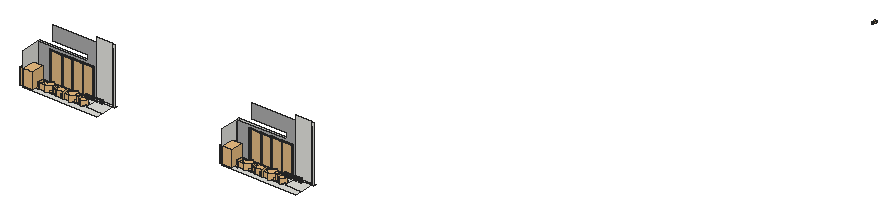
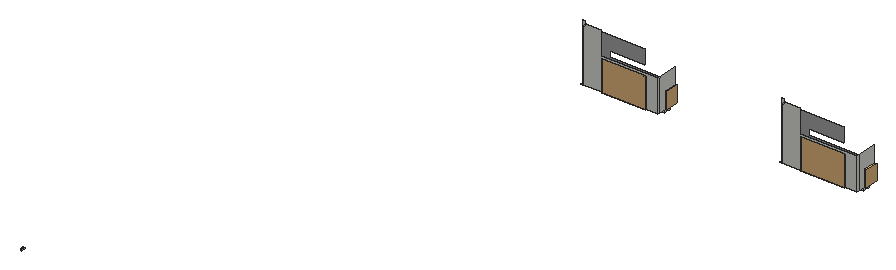
# SketchUp Ruby script. Lengths in inches.
U = 1.inch
M = Sketchup.active_model
def pt(a) = Geom::Point3d.new(a.map { |v| v * U })
def face(e, loops, mat)
  f = e.add_face(loops[0].map { |a| pt(a) })
  loops[1..].each { |l| e.add_face(l.map { |a| pt(a) }).erase! }
  f.material = f.back_material = mat if mat
  f
end
# faces: each face lists its corners as indices into pts; further lists are holes
def faces(e, pts, list, mat = nil) = list.each { |f| face(e, (f[0].is_a?(Array) ? f : [f]).map { |l| l.map { |i| pts[i] } }, mat) }
# xy, xz, yz: faces in a plane at the given z, y or x. An outline is a flat list of corners, or four numbers for a rectangle; further outlines are holes
def ring(l) = l.size == 4 ? [[l[0], l[1]], [l[2], l[1]], [l[2], l[3]], [l[0], l[3]]] : l.each_slice(2).to_a
def flat(e, list, mat, &to3) = list.each { |f| face(e, (f[0].is_a?(Array) ? f : [f]).map { |l| ring(l).map { |u, v| to3.(u, v) } }, mat) }
def xy(e, z, list, mat = nil) = flat(e, list, mat) { |x, y| [x, y, z] }
def xz(e, y, list, mat = nil) = flat(e, list, mat) { |x, z| [x, y, z] }
def yz(e, x, list, mat = nil) = flat(e, list, mat) { |y, z| [x, y, z] }
def lines(e, pts, list) = list.each { |a, b| e.add_line(pt(pts[a]), pt(pts[b])) }
# prism: a flat outline (further loops are holes) pulled along v
def prism(e, loops, v, mat = nil)
  f = face(e, loops, mat); d = Geom::Vector3d.new(v.map { |x| x * U })
  f.pushpull(f.normal.samedirection?(d) ? d.length : -d.length)
end
def box(e, o, s, mat = nil) = prism(e, [[o, [o[0] + s[0], o[1], o[2]], [o[0] + s[0], o[1] + s[1], o[2]], [o[0], o[1] + s[1], o[2]]]], [0, 0, s[2]], mat)
def at(x, y, z, deg = 0) = Geom::Transformation.translation(pt([x, y, z])) * Geom::Transformation.rotation(ORIGIN, Z_AXIS, deg.degrees)
def axes(o, x, y, z) = Geom::Transformation.new([*x, 0, *y, 0, *z, 0, *pt(o).to_a, 1])
def part(name) = M.definitions.add(name)
# library, detail: a bought-in or finely detailed component or shape, given as its bounding box
def library(name, o, s) = part(name).tap { |d| box(d.entities, o, s) }
def detail(e, o, s) = box(e.add_group.entities, o, s)
def put(e, d, t, mat = nil) = e.add_instance(d, t).tap { |i| i.material = mat if mat }
def group(e, t, mat = nil) = e.add_group.tap { |g| g.transformation = t; g.material = mat if mat }.entities
root = M.entities
M.materials.add("Glazing").color = [128, 128, 128]
M.materials["Glazing"].alpha = 0.05
M.materials.add("Material__1").color = [95, 70, 46]
M.materials.add("Powdercoating").color = [41, 44, 40]
M.materials.add("[Color M03]1").color = [170, 170, 170]
c1 = library("plant (1)",[-35.72,-28.42,0],[66.31,67.39,84.38])
c2 = library("Areca palm plant",[0,0,0],[49.1,36.6,54.46])
c3 = library("Group\#589",[-84.69,-90.07,-0.36],[176.51,175.13,171.4])
c4 = library("Group20\#1",[-20.81,-17.08,3.79],[39.86,39.43,37.51])
c5 = library("Group38\#1",[14.01,28.44,-23.43],[18.58,18.32,38.89])
c6 = library("Group\#590",[-7.34,-1.2,0],[38.67,35.81,49.04])
c7 = part("Group\#592")
put(c7.entities,c2,axes([-6.2,56.6,6.08],[0.45017,-0.56191,0],[0.66137,0.52986,0],[0,0,0.72]))
put(c7.entities,c2,axes([-6.2,158.41,6.08],[0.45017,-0.56191,0],[0.66137,0.52986,0],[0,0,0.72]))
put(c7.entities,c3,axes([17.19,15.79,6.07],[-0.08133,-0.14087,0],[0.14087,-0.08133,0],[0,0,0.1725]))
put(c7.entities,c4,axes([18.97,79.98,4.77],[0,0.85,0],[-0.85,0,0],[0,0,0.85]))
put(c7.entities,c5,axes([-4.1,-1.15,28.17],[0.8848,0,0],[0,0.94674,0],[0,0,0.85826]))
put(c7.entities,c3,axes([17.19,121.23,6.07],[-0.08133,-0.14087,0],[0.14087,-0.08133,0],[0,0,0.1725]))
put(c7.entities,c3,axes([14.93,91.37,6.05],[-0.04961,-0.08593,0],[0.08593,-0.04961,0],[0,0,0.10522]))
put(c7.entities,c4,axes([18.97,181.79,4.77],[0,0.85,0],[-0.85,0,0],[0,0,0.85]))
put(c7.entities,c3,axes([14.93,193.18,6.05],[-0.04961,-0.08593,0],[0.08593,-0.04961,0],[0,0,0.10522]))
put(c7.entities,c5,axes([-4.1,100.66,28.17],[0.8848,0,0],[0,0.94674,0],[0,0,0.85826]))
g1 = group(c7.entities,at(0,0,0))
xy(g1,0,[[0,0,6,234.8],[30,0,36,234.8]])
xy(g1,3,[[6,0,30,234.8]])
xy(g1,7,[[6,5,30,229.8]],"Material__1")
xy(g1,15,[[[0,0,36,234.8],[6,5,30,229.8]]])
xz(g1,0,[[0,0,6,0,6,3,30,3,30,0,36,0,36,15,0,15]])
xz(g1,5,[[6,7,30,15]])
xz(g1,229.8,[[6,7,30,15]])
xz(g1,234.8,[[0,0,0,15,36,15,36,0,30,0,30,3,6,3,6,0]])
yz(g1,0,[[0,0,234.8,15]])
yz(g1,6,[[0,0,234.8,3],[5,7,229.8,15]])
yz(g1,30,[[0,0,234.8,3],[5,7,229.8,15]])
yz(g1,36,[[0,0,234.8,15]])
put(c7.entities,c3,axes([17.19,223.04,6.07],[-0.08133,-0.14087,0],[0.14087,-0.08133,0],[0,0,0.1725]))
put(c7.entities,c3,axes([14.93,44.05,6.05],[-0.04961,-0.08593,0],[0.08593,-0.04961,0],[0,0,0.10522]))
put(c7.entities,c3,axes([14.93,173.12,6.05],[-0.04961,-0.08593,0],[0.08593,-0.04961,0],[0,0,0.10522]))
put(c7.entities,c3,axes([14.93,145.87,6.05],[-0.04961,-0.08593,0],[0.08593,-0.04961,0],[0,0,0.10522]))
put(c7.entities,c6,axes([24.9375,89.91,8],[0,0.79,0],[-0.79,0,0],[0,0,0.79]))
put(c7.entities,c3,axes([14.93,71.3,6.05],[-0.04961,-0.08593,0],[0.08593,-0.04961,0],[0,0,0.10522]))
put(c7.entities,c6,axes([24.9375,191.72,8],[0,0.79,0],[-0.79,0,0],[0,0,0.79]))
c8 = part("Group\#15")
xy(c8.entities,0,[[0,-55.94,0.71,45.94]])
xy(c8.entities,0.2,[[0,-55.94,0.47,45.94],[0.47,45.94,0.71,46.42]])
xy(c8.entities,2.36,[[0.47,-55.94,0.71,46.42]])
xz(c8.entities,-55.94,[[0,0,0.71,0,0.71,2.36,0.47,2.36,0.47,0.2,0,0.2]])
xz(c8.entities,45.94,[[0,0,0.71,0.2]])
xz(c8.entities,46.42,[[0.47,0.2,0.71,2.36]])
yz(c8.entities,0,[[-55.94,0,45.94,0.2]])
yz(c8.entities,0.47,[[-55.94,0.2,46.42,2.36]])
yz(c8.entities,0.71,[[-55.94,0,45.94,0,45.94,0.2,46.42,0.2,46.42,2.36,-55.94,2.36]])
c9 = part("Group\#7")
xy(c9.entities,0,[[0,-59.09,0.71,45.94]])
xy(c9.entities,0.2,[[0,-59.09,0.47,45.94],[0.47,45.94,0.71,46.42]])
xy(c9.entities,2.36,[[0.47,-59.09,0.71,46.42]])
xz(c9.entities,-59.09,[[0,0,0.71,0,0.71,2.36,0.47,2.36,0.47,0.2,0,0.2]])
xz(c9.entities,45.94,[[0,0,0.71,0.2]])
xz(c9.entities,46.42,[[0.47,0.2,0.71,2.36]])
yz(c9.entities,0,[[-59.09,0,45.94,0.2]])
yz(c9.entities,0.47,[[-59.09,0.2,46.42,2.36]])
yz(c9.entities,0.71,[[-59.09,0,45.94,0,45.94,0.2,46.42,0.2,46.42,2.36,-59.09,2.36]])
c10 = part("Group\#16")
prism(c10.entities,[[[0.47,-56.18,0.2],[0,-56.18,0.2],[0,-56.18,0],[0.71,-56.18,0],[0.71,-56.18,2.36],[0.47,-56.18,2.36]]],[0,28.68,0])
c11 = part("Group\#10")
box(c11.entities,[-0.73,0,0],[27.99,0.55,102.05])
c12 = part("Group\#18")
xy(c12.entities,0,[[0.47,-56.18,0.47,-55.47,0,-55.47,0,-28.21,1.18,-28.21,1.18,-56.18]])
xy(c12.entities,0.2,[[0.71,-56.18,1.18,-28.21],[0,-55.47,0.47,-28.21],[0.47,-28.21,0.71,-27.74]])
xy(c12.entities,2.36,[[0.47,-56.18,0.71,-27.74]])
xz(c12.entities,-56.18,[[0.47,0,1.18,0,1.18,0.2,0.71,0.2,0.71,2.36,0.47,2.36]])
xz(c12.entities,-55.47,[[0,0,0.47,0.2]])
xz(c12.entities,-28.21,[[0,0,1.18,0.2]])
xz(c12.entities,-27.74,[[0.47,0.2,0.71,2.36]])
yz(c12.entities,0,[[-55.47,0,-28.21,0.2]])
yz(c12.entities,0.47,[[-56.18,0,-55.47,0.2],[-56.18,0.2,-27.74,2.36]])
yz(c12.entities,0.71,[[-56.18,0.2,-27.74,2.36]])
yz(c12.entities,1.18,[[-56.18,0,-28.21,0.2]])
c13 = part("Group\#34")
xy(c13.entities,0,[[-20.45,0,7.76,1.22]])
xy(c13.entities,0.06,[[-20.39,0.06,7.7,1.22]])
xy(c13.entities,0.47,[[-19.98,0,7.28,0.06]])
xy(c13.entities,101.89,[[-19.98,0,7.28,0.06]])
xy(c13.entities,102.3,[[-20.39,0.06,7.7,1.22]])
xy(c13.entities,102.36,[[-20.45,0,7.76,1.22]])
xz(c13.entities,0,[[[-20.45,0,7.76,102.36],[-19.98,0.47,7.28,101.89]]])
xz(c13.entities,0.06,[[[-20.39,0.06,7.7,102.3],[-19.98,0.47,7.28,101.89]]])
xz(c13.entities,1.22,[[[-20.45,0,7.76,102.36],[-20.39,0.06,7.7,102.3]]])
yz(c13.entities,-20.45,[[0,0,1.22,102.36]])
yz(c13.entities,-20.39,[[0.06,0.06,1.22,102.3]])
yz(c13.entities,-19.98,[[0,0.47,0.06,101.89]])
yz(c13.entities,7.28,[[0,0.47,0.06,101.89]])
yz(c13.entities,7.7,[[0.06,0.06,1.22,102.3]])
yz(c13.entities,7.76,[[0,0,1.22,102.36]])
c14 = part("Group\#6")
put(c14.entities,c8,axes([27.97,0,7.875],[1,0,0],[0,0,-1],[0,1,0]),"Powdercoating")
put(c14.entities,c9,axes([0.71,0,6.8],[-1,0,0],[0,0,-0.97687],[0,1,0]),"Powdercoating")
put(c14.entities,c10,axes([-27.5,0,-38.07],[0,0,-1],[-1,0,0],[0,1,0]),"Powdercoating")
put(c14.entities,c11,at(1.12,0.35,-38.39),"Glazing")
put(c14.entities,c12,axes([-27.5,0,63.35],[0,0,1],[-1,0,0],[0,1,0]),"Powdercoating")
put(c14.entities,c13,at(20.6875,1.0625,-38.54),"Powdercoating")
c15 = part("Component\#2")
put(c15.entities,c14,at(-1.18,4.5,38.86))
g2 = group(c15.entities,at(84.74,4.5,38.86))
put(g2,c8,axes([-27.97,0,7.875],[-1,0,0],[0,0,-1],[0,1,0]),"Powdercoating")
put(g2,c9,axes([-0.71,0,6.8],[1,0,0],[0,0,-0.97687],[0,1,0]),"Powdercoating")
put(g2,c10,axes([27.5,0,-38.07],[0,0,-1],[1,0,0],[0,1,0]),"Powdercoating")
put(g2,c11,axes([-1.12,0.35,-38.39],[-1,0,0],[0,1,0],[0,0,1]),"Glazing")
put(g2,c12,axes([27.5,0,63.35],[0,0,1],[1,0,0],[0,1,0]),"Powdercoating")
put(g2,c13,axes([-20.6875,1.0625,-38.54],[-1,0,0],[0,1,0],[0,0,1]),"Powdercoating")
g3 = group(c15.entities,at(56.0625,4.5,38.86))
put(g3,c8,axes([-27.97,0,7.875],[-1,0,0],[0,0,-1],[0,1,0]),"Powdercoating")
put(g3,c10,axes([27.5,0,-38.07],[0,0,-1],[1,0,0],[0,1,0]),"Powdercoating")
put(g3,c11,axes([-1.12,0.35,-38.39],[-1,0,0],[0,1,0],[0,0,1]),"Glazing")
put(g3,c12,axes([27.5,0,63.35],[0,0,1],[1,0,0],[0,1,0]),"Powdercoating")
put(g3,c13,axes([-20.6875,1.0625,-38.54],[-1,0,0],[0,1,0],[0,0,1]),"Powdercoating")
g4 = group(g3,at(-0.71,0,6.8),"Powdercoating")
xy(g4,-45.34,[[0.47,0.2,0.71,2.36]])
xy(g4,-44.88,[[0,0,0.71,0.2]])
xy(g4,57.73,[[0,0,0.71,0,0.71,2.36,0.47,2.36,0.47,0.2,0,0.2]])
xz(g4,0,[[0,-44.88,0.71,57.73]])
xz(g4,0.2,[[0.47,-45.34,0.71,-44.88],[0,-44.88,0.47,57.73]])
xz(g4,2.36,[[0.47,-45.34,0.71,57.73]])
yz(g4,0,[[0,-44.88,0.2,57.73]])
yz(g4,0.47,[[0.2,-45.34,2.36,57.73]])
yz(g4,0.71,[[0.2,-45.34,2.36,-45.34,2.36,57.73,0,57.73,0,-44.88,0.2,-44.88]])
put(c15.entities,c14,axes([-33.94,4.5,38.86],[1.14218,0,0],[0,1,0],[0,0,1]))
c16 = part("sliding door")
put(c16.entities,c15,at(0,-4.5,-0.08))
c17 = library("panneau+shadow+blanc+bourdon+naturel",[-47.99,-1.29,1.53],[97.82,5.86,114.18])
c18 = library("Group\#544",[0,0,0],[9.97,16.11,7.56])
xy(root,203.4375,[[227.71,1092.87,620.51,1092.87,620.51,1125.04,533.89,1125.04,533.89,1194.07,227.71,1194.07],[1276.02,1092.87,1668.82,1092.87,1668.82,1125.04,1582.21,1125.04,1582.21,1194.07,1276.02,1194.07],[533.89,1125.04,620.51,1194.07],[1582.21,1125.04,1668.82,1194.07],[227.71,1194.07,292.46,1206.01],
  [292.46,1194.07,519.89,1206.01],[519.89,1194.07,620.51,1206.01],[620.51,1194.07,632.45,1206.01],[1276.02,1194.07,1340.77,1206.01],[1340.77,1194.07,1568.21,1206.01],
  [1568.21,1194.07,1668.82,1206.01],[1668.82,1194.07,1680.76,1206.01]])
xz(root,1127.73,[[1582.21,242.84,1668.82,243.875],[533.89,246.91,620.51,247.9375],[1582.21,246.91,1668.82,247.9375],[533.89,250.97,620.51,252],[1582.21,250.97,1668.82,252],
  [533.89,255.03,620.51,256.0625],[1582.21,255.03,1668.82,256.0625],[533.89,259.09,620.51,260.125],[1582.21,259.09,1668.82,260.125],[533.89,263.16,620.51,264.1875],
  [1582.21,263.16,1668.82,264.1875]])
xz(root,1194.07,[[620.51,203.4375,632.45,500.5],[1668.82,203.4375,1680.76,500.5]])
xz(root,1194.07,[[227.71,203.4375,292.46,203.4375,292.46,360.0625,519.89,360.0625,519.89,203.4375,533.89,203.4375,533.89,480,308.31,480,308.31,404.4375,490.65,404.4375,490.65,375.08,227.71,375.08],[1276.02,203.4375,1340.77,203.4375,1340.77,360.0625,1568.21,360.0625,1568.21,203.4375,1582.21,203.4375,1582.21,480,1356.62,480,1356.62,404.4375,1538.96,404.4375,1538.96,375.08,1276.02,375.08]],"[Color M03]1")
xz(root,1206.01,[[227.71,203.4375,227.71,375.08,528.02,375.08,528.02,495.5,609,495.5,609,482.53,620.51,482.53,620.51,203.4375,519.89,203.4375,519.89,360.0625,292.46,360.0625,292.46,203.4375],[1276.02,203.4375,1276.02,375.08,1576.34,375.08,1576.34,495.5,1657.31,495.5,1657.31,482.53,1668.82,482.53,1668.82,203.4375,1568.21,203.4375,1568.21,360.0625,1340.77,360.0625,1340.77,203.4375]])
yz(root,227.71,[[1092.87,203.4375,1194.07,375.08],[1194.07,203.4375,1206.01,375.08]])
yz(root,292.46,[[1194.07,203.4375,1206.01,360.0625]])
yz(root,519.89,[[1194.07,203.4375,1206.01,360.0625]])
yz(root,620.51,[[1194.07,203.4375,1206.01,482.53]])
yz(root,1276.02,[[1092.87,203.4375,1194.07,375.08],[1194.07,203.4375,1206.01,375.08]])
yz(root,1340.77,[[1194.07,203.4375,1206.01,360.0625]])
yz(root,1568.21,[[1194.07,203.4375,1206.01,360.0625]])
yz(root,1668.82,[[1194.07,203.4375,1206.01,482.53]])
put(root,c1,at(250.6,1122.52,210.17))
put(root,c1,at(1298.91,1122.52,210.17))
put(root,c7,axes([524.03,1125.04,189.375],[0,1,0],[-1.25931,0,0],[0,0,1]))
put(root,c7,axes([1572.34,1125.04,189.375],[0,1,0],[-1.25931,0,0],[0,0,1]))
put(root,c16,axes([357.21,1191.74,203.14],[1.9177,0,0],[0,1.51,0],[0,0,1.51]))
put(root,c16,axes([1405.52,1191.74,203.14],[1.9177,0,0],[0,1.51,0],[0,0,1.51]))
put(root,c17,axes([404.04,1202.43,201.33],[2.32508,0,0],[0,1,0],[0,0,1.37182]))
put(root,c17,axes([1452.35,1202.43,201.33],[2.32508,0,0],[0,1,0],[0,0,1.37182]))
put(root,c18,at(2611.13,3705.92,194.01))
